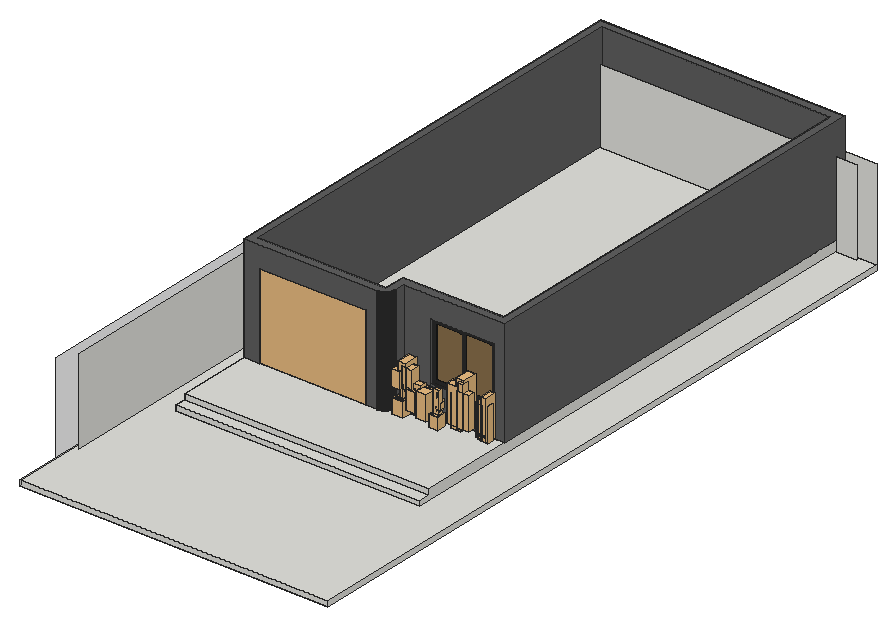
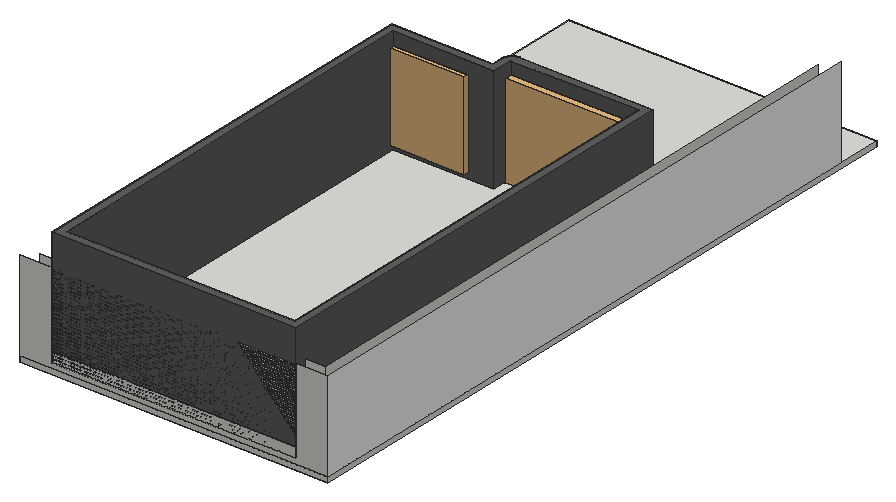
# SketchUp Ruby script. Lengths in inches.
U = 1.inch
M = Sketchup.active_model
def pt(a) = Geom::Point3d.new(a.map { |v| v * U })
def face(e, loops, mat)
  f = e.add_face(loops[0].map { |a| pt(a) })
  loops[1..].each { |l| e.add_face(l.map { |a| pt(a) }).erase! }
  f.material = f.back_material = mat if mat
  f
end
# faces: each face lists its corners as indices into pts; further lists are holes
def faces(e, pts, list, mat = nil) = list.each { |f| face(e, (f[0].is_a?(Array) ? f : [f]).map { |l| l.map { |i| pts[i] } }, mat) }
# xy, xz, yz: faces in a plane at the given z, y or x. An outline is a flat list of corners, or four numbers for a rectangle; further outlines are holes
def ring(l) = l.size == 4 ? [[l[0], l[1]], [l[2], l[1]], [l[2], l[3]], [l[0], l[3]]] : l.each_slice(2).to_a
def flat(e, list, mat, &to3) = list.each { |f| face(e, (f[0].is_a?(Array) ? f : [f]).map { |l| ring(l).map { |u, v| to3.(u, v) } }, mat) }
def xy(e, z, list, mat = nil) = flat(e, list, mat) { |x, y| [x, y, z] }
def xz(e, y, list, mat = nil) = flat(e, list, mat) { |x, z| [x, y, z] }
def yz(e, x, list, mat = nil) = flat(e, list, mat) { |y, z| [x, y, z] }
def lines(e, pts, list) = list.each { |a, b| e.add_line(pt(pts[a]), pt(pts[b])) }
# prism: a flat outline (further loops are holes) pulled along v
def prism(e, loops, v, mat = nil)
  f = face(e, loops, mat); d = Geom::Vector3d.new(v.map { |x| x * U })
  f.pushpull(f.normal.samedirection?(d) ? d.length : -d.length)
end
def box(e, o, s, mat = nil) = prism(e, [[o, [o[0] + s[0], o[1], o[2]], [o[0] + s[0], o[1] + s[1], o[2]], [o[0], o[1] + s[1], o[2]]]], [0, 0, s[2]], mat)
def at(x, y, z, deg = 0) = Geom::Transformation.translation(pt([x, y, z])) * Geom::Transformation.rotation(ORIGIN, Z_AXIS, deg.degrees)
def axes(o, x, y, z) = Geom::Transformation.new([*x, 0, *y, 0, *z, 0, *pt(o).to_a, 1])
def part(name) = M.definitions.add(name)
# library, detail: a bought-in or finely detailed component or shape, given as its bounding box
def library(name, o, s) = part(name).tap { |d| box(d.entities, o, s) }
def detail(e, o, s) = box(e.add_group.entities, o, s)
def put(e, d, t, mat = nil) = e.add_instance(d, t).tap { |i| i.material = mat if mat }
def group(e, t, mat = nil) = e.add_group.tap { |g| g.transformation = t; g.material = mat if mat }.entities
root = M.entities
M.materials.add("1421 AP 8232 ELEGANT GREY").color = [96, 96, 96]
M.materials.add("BANANA_BIG_STVOL_1").color = [93, 83, 53]
M.materials.add("Glass_Tinted_Gray").color = [0, 0, 0]
M.materials["Glass_Tinted_Gray"].alpha = 0.125
M.materials.add("POT_TEXTURE_2").color = [160, 154, 144]
M.materials.add("[0135_DarkGray]").color = [81, 81, 81]
M.materials.add("[Metal Seamed]").color = [36, 36, 35]
M.materials.add("[Mirror 02]").color = [229, 229, 229]
M.materials.add("[Quartz Light Grey]").color = [251, 251, 252]
M.materials.add("[Terrazzo Light Blue]").color = [196, 214, 227]
M.materials.add("soil1").color = [68, 55, 47]
M.materials.add("white_concrete_pot1").color = [212, 211, 204]
M.materials.add("wood_1").color = [140, 119, 94]
c1 = library("Group\#110",[-310.7,1952.62,354.63],[79.53,58.52,39.48])
c2 = library("Group\#213",[-330.26,-2159.14,612.04],[116.66,119.22,673.97])
c3 = library("Group\#85",[-312.76,2118.02,370.79],[80.37,61.43,57.53])
c4 = library("Group\#192",[-513.94,-1201.2,195.17],[480.66,557.42,1160.08])
c5 = library("Group\#163",[-447.02,-464.95,536.35],[343.73,346.24,39.39])
c6 = library("Group\#189",[-492.14,-508.4,-4.15],[433.72,431.71,567.03])
c7 = library("Group\#129",[-315.77,2202.04,371],[80.74,54.44,37.85])
c8 = library("Group\#206",[-390.1,-1177.12,195.59],[220.93,265.44,790.12])
c9 = library("Group\#210",[-480.3,-2300.47,677.45],[398.14,398.43,28.25])
c10 = library("Group\#217",[-568.09,-2386.9,-3.76],[573.62,569.18,700.28])
c11 = library("Group\#160",[-455.56,899.32,410.78],[341.21,610.33,1581.5])
c12 = library("Group\#104",[-330.83,2117.69,370.2],[61.83,80.2,35.55])
c13 = library("Group\#109",[-340.96,1970.4,361.28],[81.22,51.59,61.62])
c14 = library("Group\#154",[-445.29,890.31,329.28],[284.3,304.08,2023.29])
c15 = library("Group\#188",[-385.21,-446.52,494.02],[160.93,321.12,1142.36])
c16 = library("Group\#173",[-341.93,-403.49,744.8125],[64.83,96.32,132.15])
c17 = library("Group\#205",[-445.7,-1606.55,154.18],[255.44,283.57,849.28])
c18 = library("Group\#120",[-363.89,1895.22,354.63],[76.92,66.54,39.48])
c19 = library("Group\#135",[-366.3125,2177.8,359.41],[79.9,61.23,37.86])
c20 = library("Group\#186",[-422.77,-235.4,843.61],[178.54,197.77,233.54])
c21 = library("Group\#131",[-372.4375,2154.5,374],[76.125,67.08,39.0625])
c22 = library("Group\#102",[-362.86,1963.26,351.01],[55.56,80.44,37.9])
c23 = library("Group\#193",[-545.36,-1775.03,287.125],[412.21,432,920.68])
c24 = library("Group\#177",[-388.93,-514.39,838.93],[89.79,77.73,82.08])
c25 = library("Group\#174",[-424,-312.27,817.53],[158.81,108.06,136.45])
c26 = library("Group\#96",[-374.28,1979.7,369.99],[51.81,82.66,37.9])
c27 = library("Group\#164",[-394.9,-448.99,911.74],[90.19,96.88,85.93])
c28 = library("Group\#121",[-390.04,2074.71,363.78],[77.3,84.83,61.55])
c29 = library("Group\#94",[-392.38,2142.99,345.23],[79.77,60.6,39.05])
c30 = library("Group\#167",[-438.92,-265.61,702.3],[171.52,146.16,133.5])
c31 = library("Group\#98",[-389.63,2051.04,359.41],[56.81,81.38,37.86])
c32 = library("Group\#127",[-397.18,1916.74,372.44],[70.02,74.57,49.25])
c33 = library("Group\#219",[-550.09,-2664.39,1031.96],[371.42,533.86,798])
c34 = library("Group\#178",[-409.02,-515.05,915.53],[69.62,77.27,65.47])
c35 = library("Group\#122",[-419.21,1941.11,355.02],[73.1,71.21,39.06])
c36 = library("Group\#143",[-527.15,2088.47,150.96],[267.01,328.12,1599.25])
c37 = library("Group\#169",[-545.09,-386.51,922.3125],[300.25,219.65,227.33])
c38 = library("Group\#95",[-433.57,2042.61,369.7],[71.79,72.8,37.85])
c39 = library("Group\#97",[-432.01,1984.38,372.6875],[64.1,75.95,39.0625])
c40 = library("Group\#101",[-435.875,2067.96,347.82],[58.32,80.53,38.29])
c41 = library("Group\#176",[-568.91,-444.37,1285.4],[307.6,179.39,277.93])
c42 = library("Group\#140",[-571.16,1736.08,232.33],[294.08,306.57,1438.75])
c43 = library("Group\#180",[-498.98,-524.4,908.45],[120.83,107.95,112.98])
c44 = library("Group\#197",[-640.625,-1318.37,287.11],[396.64,314.81,689.96])
c45 = library("Group\#148",[-616.67,2098.6,178.29],[331.19,111.16,1177.92])
c46 = library("Group\#214",[-667.53,-2111.4375,1071.74],[420.02,555.28,968.03])
c47 = library("Group\#200",[-619.83,-1636.3,288.9],[316.15,456.61,1171.28])
c48 = library("Group\#159",[-662.41,217.3,320.04],[397.32,658.3,1732.06])
c49 = library("Group\#144",[-675.58,1862.05,152.55],[378.81,196.01,1743.84])
c50 = library("Group\#157",[-733.48,439.625,202.64],[456.28,533.12,1536.78])
c51 = library("Group\#150",[-792.12,2067.32,152.13],[549.56,259.52,1931.8])
c52 = library("Group\#201",[-738.91,-1210.08,301],[426.4,388.88,1000.79])
c53 = library("Group\#198",[-750.24,-1478.51,301.56],[423.84,451.05,998.69])
c54 = library("Group\#138",[-904.81,1865.01,156.3],[624.43,217.34,1227.7])
c55 = library("Group\#216",[-943.22,-2312.1875,967.59],[670.63,402.45,1245.73])
c56 = library("Group\#156",[-1038.76,656.55,345.34],[733.18,460.51,2065.7])
c57 = library("Curtain assembly",[0,0,0],[57.48,5.46,98.43])
c58 = library("Curtains",[0,0,0],[121.73,8.19,117.22])
c59 = library("Group\#3",[0,-4.26,0],[120,5.53,96])
c60 = part("PENTEK_RP Fineline 50S_Sliding_DoorCase_E1")
box(c60.entities,[0,0,0],[1.51,3.66,99.27],"[0135_DarkGray]")
c61 = part("PENTEK_RP Fineline 50S_SlidingDooe_Case_E2")
box(c61.entities,[0,0,0],[96.25,3.66,1.51],"[0135_DarkGray]")
c62 = part("pentek_RP Fineline 50S_SlidingDoor_Case")
put(c62.entities,c60,at(97.76,0,0))
put(c62.entities,c61,at(1.51,0,0))
put(c62.entities,c60,at(0,0,0),"[Metal Seamed]")
put(c62.entities,c61,at(1.51,0,97.76),"[Metal Seamed]")
c63 = part("PENTEK_RP Fineline 50S_SlidingDoor_GlazingBead_2")
box(c63.entities,[0,0,0],[0.56,0.59,94.39],"[0135_DarkGray]")
c64 = part("PENTEK_RP Fineline 50S_SlidingDoor_Glass")
box(c64.entities,[0,0,0],[46.58,0.16,94.39],"Glass_Tinted_Gray")
c65 = part("PENTEK_RP Fineline 50S_SlidingDoor_GlazingBead")
box(c65.entities,[0,0,0],[45.47,0.59,0.56],"[0135_DarkGray]")
c66 = part("PENTEK_RP Fineline 50S_SlidingDoor_Leaf_E1")
xy(c66.entities,0,[[0,0,0.93,1.97],[0.93,1.57,1.49,1.97]],"[0135_DarkGray]")
xy(c66.entities,96.25,[[0,0,0.93,0,0.93,1.57,1.49,1.57,1.49,1.97,0,1.97]],"[0135_DarkGray]")
xz(c66.entities,0,[[0,0,0.93,96.25]],"[0135_DarkGray]")
xz(c66.entities,1.57,[[0.93,0,1.49,95.32],[0.93,95.32,1.49,96.25]],"[0135_DarkGray]")
xz(c66.entities,1.97,[[0,0,1.49,96.25]],"[0135_DarkGray]")
yz(c66.entities,0,[[0,0,1.97,96.25]],"[0135_DarkGray]")
yz(c66.entities,0.93,[[0,0,1.57,0.93],[0,0.93,1.57,95.32],[0,95.32,1.57,96.25]],"[0135_DarkGray]")
yz(c66.entities,1.49,[[1.57,0,1.97,95.32],[1.57,95.32,1.97,96.25]],"[0135_DarkGray]")
c67 = part("PENTEK_RP Fineline 50S_SlidingDoor_Leaf_E2")
xy(c67.entities,0,[[0,0,0,1.57,0.56,1.57,0.56,1.97,46.02,1.97,46.02,1.57,46.58,1.57,46.58,0]],"[0135_DarkGray]")
xy(c67.entities,0.93,[[0,0,46.58,1.57]],"[0135_DarkGray]")
xy(c67.entities,1.49,[[0.56,1.57,46.02,1.97]],"[0135_DarkGray]")
xz(c67.entities,0,[[0,0,46.58,0.93]],"[0135_DarkGray]")
xz(c67.entities,1.57,[[0,0,0.56,0.93],[46.02,0,46.58,0.93],[0.56,0.93,46.02,1.49]],"[0135_DarkGray]")
xz(c67.entities,1.97,[[0.56,0,46.02,1.49]],"[0135_DarkGray]")
yz(c67.entities,0,[[0,0,1.57,0.93]],"[0135_DarkGray]")
yz(c67.entities,0.56,[[1.57,0,1.97,0.93],[1.57,0.93,1.97,1.49]],"[0135_DarkGray]")
yz(c67.entities,46.02,[[1.57,0,1.97,0.93],[1.57,0.93,1.97,1.49]],"[0135_DarkGray]")
yz(c67.entities,46.58,[[0,0,1.57,0.93]],"[0135_DarkGray]")
c68 = part("PENTEK_RP Fineline S_SlidingDoor_Leaf1")
put(c68.entities,c63,at(0.93,0,0.93))
put(c68.entities,c63,at(46.96,0,0.93))
put(c68.entities,c64,at(1.49,1.42,0.93))
put(c68.entities,c65,at(1.49,0,0.93))
put(c68.entities,c64,at(1.49,0.59,0.93),"[Terrazzo Light Blue]")
put(c68.entities,c66,at(0,0,0))
put(c68.entities,c66,axes([48.44,0,0],[-1,0,0],[0,1,0],[0,0,1]))
put(c68.entities,c67,axes([0.93,0,96.25],[1,0,0],[0,1,0],[0,0,-1]))
put(c68.entities,c67,at(0.93,0,0))
put(c68.entities,c65,at(1.49,0,94.77))
c69 = part("PENTEK_RP Fineline 50S_SlidingDoor_Leaf2")
put(c69.entities,c64,at(1.49,1.42,0.93))
put(c69.entities,c65,at(1.49,0,94.77))
put(c69.entities,c63,at(46.96,0,0.93))
put(c69.entities,c64,at(1.49,0.59,0.93),"[Mirror 02]")
put(c69.entities,c63,at(0.93,0,0.93))
put(c69.entities,c66,at(0,0,0))
put(c69.entities,c66,axes([48.44,0,0],[-1,0,0],[0,1,0],[0,0,1]))
put(c69.entities,c65,at(1.49,0,0.93))
put(c69.entities,c67,axes([0.93,0,96.25],[1,0,0],[0,1,0],[0,0,-1]))
put(c69.entities,c67,at(0.93,0,0))
c70 = part("PENTEK - Slimmest Steel Sliding Door / Window\#1")
put(c70.entities,c62,at(0,-1.88,-0.09))
put(c70.entities,c68,at(1.51,-2.27,1.42))
put(c70.entities,c69,at(49.32,-0.3,1.42))
xz(root,763,[[12,-12,336,84]])
xz(root,775,[[0,-18,348,84]])
yz(root,0,[[50,-18,775,84]],"[Quartz Light Grey]")
yz(root,12,[[67,-12,763,84]])
put(root,c1,axes([253.68,273.14,0.11],[0,-0.02318,0],[0.02157,0,0],[0,0,0.02333]),"white_concrete_pot1")
put(root,c2,axes([253.68,273.14,0.11],[0,-0.02318,0],[0.02157,0,0],[0,0,0.02333]),"BANANA_BIG_STVOL_1")
put(root,c3,axes([253.68,273.14,0.11],[0,-0.02318,0],[0.02157,0,0],[0,0,0.02333]),"white_concrete_pot1")
put(root,c4,axes([253.68,273.14,0.11],[0,-0.02318,0],[0.02157,0,0],[0,0,0.02333]))
put(root,c5,axes([253.68,273.14,0.11],[0,-0.02318,0],[0.02157,0,0],[0,0,0.02333]),"soil1")
put(root,c6,axes([253.68,273.14,0.11],[0,-0.02318,0],[0.02157,0,0],[0,0,0.02333]),"POT_TEXTURE_2")
put(root,c7,axes([253.68,273.14,0.11],[0,-0.02318,0],[0.02157,0,0],[0,0,0.02333]),"white_concrete_pot1")
g1 = group(root,at(253.68,273.14,0.11),"white_concrete_pot1")
detail(g1,[40.58,5.65,8.19],[1.57,1.63,0.87])
put(root,c8,axes([253.68,273.14,0.11],[0,-0.02318,0],[0.02157,0,0],[0,0,0.02333]))
put(root,c9,axes([253.68,273.14,0.11],[0,-0.02318,0],[0.02157,0,0],[0,0,0.02333]),"soil1")
put(root,c10,axes([253.68,273.14,0.11],[0,-0.02318,0],[0.02157,0,0],[0,0,0.02333]),"POT_TEXTURE_2")
g2 = group(root,at(253.68,273.14,0.11),"white_concrete_pot1")
detail(g2,[44.84,5.64,7.91],[1.49,1.76,0.92])
put(root,c11,axes([253.68,273.14,0.11],[0,-0.02318,0],[0.02157,0,0],[0,0,0.02333]))
put(root,c12,axes([253.68,273.14,0.11],[0,-0.02318,0],[0.02157,0,0],[0,0,0.02333]),"white_concrete_pot1")
put(root,c13,axes([253.68,273.14,0.11],[0,-0.02318,0],[0.02157,0,0],[0,0,0.02333]),"white_concrete_pot1")
g3 = group(root,at(253.68,273.14,0.11),"white_concrete_pot1")
detail(g3,[40.82,6.3,8.64],[1.71,1.42,0.87])
put(root,c14,axes([253.68,273.14,0.11],[0,-0.02318,0],[0.02157,0,0],[0,0,0.02333]))
put(root,c15,axes([253.68,273.14,0.11],[0,-0.02318,0],[0.02157,0,0],[0,0,0.02333]),"wood_1")
put(root,c16,axes([253.68,273.14,0.11],[0,-0.02318,0],[0.02157,0,0],[0,0,0.02333]))
put(root,c17,axes([253.68,273.14,0.11],[0,-0.02318,0],[0.02157,0,0],[0,0,0.02333]))
put(root,c18,axes([253.68,273.14,0.11],[0,-0.02318,0],[0.02157,0,0],[0,0,0.02333]),"white_concrete_pot1")
put(root,c19,axes([253.68,273.14,0.11],[0,-0.02318,0],[0.02157,0,0],[0,0,0.02333]),"white_concrete_pot1")
put(root,c20,axes([253.68,273.14,0.11],[0,-0.02318,0],[0.02157,0,0],[0,0,0.02333]))
put(root,c21,axes([253.68,273.14,0.11],[0,-0.02318,0],[0.02157,0,0],[0,0,0.02333]),"white_concrete_pot1")
put(root,c22,axes([253.68,273.14,0.11],[0,-0.02318,0],[0.02157,0,0],[0,0,0.02333]),"white_concrete_pot1")
put(root,c23,axes([253.68,273.14,0.11],[0,-0.02318,0],[0.02157,0,0],[0,0,0.02333]))
put(root,c24,axes([253.68,273.14,0.11],[0,-0.02318,0],[0.02157,0,0],[0,0,0.02333]))
put(root,c25,axes([253.68,273.14,0.11],[0,-0.02318,0],[0.02157,0,0],[0,0,0.02333]))
put(root,c26,axes([253.68,273.14,0.11],[0,-0.02318,0],[0.02157,0,0],[0,0,0.02333]),"white_concrete_pot1")
put(root,c27,axes([253.68,273.14,0.11],[0,-0.02318,0],[0.02157,0,0],[0,0,0.02333]))
put(root,c28,axes([253.68,273.14,0.11],[0,-0.02318,0],[0.02157,0,0],[0,0,0.02333]),"white_concrete_pot1")
put(root,c29,axes([253.68,273.14,0.11],[0,-0.02318,0],[0.02157,0,0],[0,0,0.02333]),"white_concrete_pot1")
put(root,c30,axes([253.68,273.14,0.11],[0,-0.02318,0],[0.02157,0,0],[0,0,0.02333]))
g4 = group(root,at(253.68,273.14,0.11),"white_concrete_pot1")
detail(g4,[43.93,7.3,8.4],[1.4,1.85,0.87])
put(root,c31,axes([253.68,273.14,0.11],[0,-0.02318,0],[0.02157,0,0],[0,0,0.02333]),"white_concrete_pot1")
put(root,c32,axes([253.68,273.14,0.11],[0,-0.02318,0],[0.02157,0,0],[0,0,0.02333]),"white_concrete_pot1")
put(root,c33,axes([253.68,273.14,0.11],[0,-0.02318,0],[0.02157,0,0],[0,0,0.02333]))
put(root,c34,axes([253.68,273.14,0.11],[0,-0.02318,0],[0.02157,0,0],[0,0,0.02333]))
put(root,c35,axes([253.68,273.14,0.11],[0,-0.02318,0],[0.02157,0,0],[0,0,0.02333]),"white_concrete_pot1")
g5 = group(root,at(253.68,273.14,0.11),"white_concrete_pot1")
detail(g5,[45.57,8.17,8.63],[1.72,1.51,0.89])
put(root,c36,axes([253.68,273.14,0.11],[0,-0.02318,0],[0.02157,0,0],[0,0,0.02333]))
put(root,c37,axes([253.68,273.14,0.11],[0,-0.02318,0],[0.02157,0,0],[0,0,0.02333]))
g6 = group(root,at(253.68,273.14,0.11),"white_concrete_pot1")
detail(g6,[43.74,8.27,8.18],[1.35,1.83,0.89])
put(root,c38,axes([253.68,273.14,0.11],[0,-0.02318,0],[0.02157,0,0],[0,0,0.02333]),"white_concrete_pot1")
put(root,c39,axes([253.68,273.14,0.11],[0,-0.02318,0],[0.02157,0,0],[0,0,0.02333]),"white_concrete_pot1")
put(root,c40,axes([253.68,273.14,0.11],[0,-0.02318,0],[0.02157,0,0],[0,0,0.02333]),"white_concrete_pot1")
put(root,c41,axes([253.68,273.14,0.11],[0,-0.02318,0],[0.02157,0,0],[0,0,0.02333]))
put(root,c42,axes([253.68,273.14,0.11],[0,-0.02318,0],[0.02157,0,0],[0,0,0.02333]))
put(root,c43,axes([253.68,273.14,0.11],[0,-0.02318,0],[0.02157,0,0],[0,0,0.02333]))
put(root,c44,axes([253.68,273.14,0.11],[0,-0.02318,0],[0.02157,0,0],[0,0,0.02333]))
put(root,c45,axes([253.68,273.14,0.11],[0,-0.02318,0],[0.02157,0,0],[0,0,0.02333]))
put(root,c46,axes([253.68,273.14,0.11],[0,-0.02318,0],[0.02157,0,0],[0,0,0.02333]))
put(root,c47,axes([253.68,273.14,0.11],[0,-0.02318,0],[0.02157,0,0],[0,0,0.02333]))
put(root,c48,axes([253.68,273.14,0.11],[0,-0.02318,0],[0.02157,0,0],[0,0,0.02333]))
put(root,c49,axes([253.68,273.14,0.11],[0,-0.02318,0],[0.02157,0,0],[0,0,0.02333]))
put(root,c50,axes([253.68,273.14,0.11],[0,-0.02318,0],[0.02157,0,0],[0,0,0.02333]))
put(root,c51,axes([253.68,273.14,0.11],[0,-0.02318,0],[0.02157,0,0],[0,0,0.02333]))
put(root,c52,axes([253.68,273.14,0.11],[0,-0.02318,0],[0.02157,0,0],[0,0,0.02333]))
put(root,c53,axes([253.68,273.14,0.11],[0,-0.02318,0],[0.02157,0,0],[0,0,0.02333]))
put(root,c54,axes([253.68,273.14,0.11],[0,-0.02318,0],[0.02157,0,0],[0,0,0.02333]))
put(root,c55,axes([253.68,273.14,0.11],[0,-0.02318,0],[0.02157,0,0],[0,0,0.02333]))
put(root,c56,axes([253.68,273.14,0.11],[0,-0.02318,0],[0.02157,0,0],[0,0,0.02333]))
g7 = group(root,at(0,0,-18))
box(g7,[0,0,-6],[348,775,6])
g8 = group(root,at(36,271,0))
prism(g8,[[[0,-84,0],[0,504,0],[0,504,-12],[0,-96,-12],[0,-96,-6],[0,-84,-6]]],[276,0,0])
g9 = group(root,at(36,295,0),"1421 AP 8232 ELEGANT GREY")
xy(g9,0,[[0,-24,0,480,276,480,276,0,162,0,162,-12.3125,161.99,-12.47,161.98,-12.63,161.97,-12.78,161.95,-13.1,161.93,-13.25,161.92,-13.41,161.9,-13.57,161.875,-13.72,161.85,-13.88,161.83,-14.03,161.8,-14.1875,161.77,-14.34,161.74,-14.49,161.7,-14.65,161.67,-14.8,161.63,-14.95,161.59,-15.11,161.51,-15.41,161.36,-15.86,161.3125,-16.01,161.26,-16.15,161.2,-16.3,161.15,-16.45,161.09,-16.59,161.03,-16.74,160.96,-16.88,160.9,-17.02,160.83,-17.17,160.55,-17.73,160.47,-17.86,160.39,-18,160.3125,-18.14,160.23,-18.27,160.15,-18.4,160.0625,-18.54,159.98,-18.67,159.8,-18.93,159.71,-19.05,159.62,-19.18,159.52,-19.31,159.42,-19.43,159.33,-19.55,159.23,-19.67,159.02,-19.91,158.92,-20.03,158.8125,-20.15,158.7,-20.26,158.6,-20.375,158.49,-20.49,158.375,-20.6,158.26,-20.7,158.15,-20.8125,158.03,-20.92,157.91,-21.02,157.67,-21.23,157.55,-21.33,157.43,-21.42,157.31,-21.52,157.18,-21.62,157.05,-21.71,156.93,-21.8,156.67,-21.98,156.54,-22.0625,156.4,-22.15,156.27,-22.23,156.14,-22.3125,156,-22.39,155.86,-22.47,155.73,-22.55,155.17,-22.83,155.02,-22.9,154.88,-22.96,154.74,-23.03,154.59,-23.09,154.45,-23.15,154.3,-23.2,154.15,-23.26,154.01,-23.3125,153.86,-23.36,153.41,-23.51,153.11,-23.59,152.95,-23.63,152.8,-23.67,152.65,-23.7,152.49,-23.74,152.34,-23.77,152.1875,-23.8,152.03,-23.83,151.88,-23.85,151.72,-23.875,151.57,-23.9,151.41,-23.92,151.25,-23.93,151.1,-23.95,150.78,-23.97,150.63,-23.98,150.47,-23.99,150.3125,-24,138,-24,138,-15,153,-15,153,9,267,9,267,471,9,471,9,-15,18,-15,18,-24]])
xy(g9,30,[[192,0,264,9]])
xy(g9,96,[[18,-24,138,-15],[192,0,264,9]])
xy(g9,120,[[[0,-24,150.3125,-24,150.47,-23.99,150.63,-23.98,150.78,-23.97,151.1,-23.95,151.25,-23.93,151.41,-23.92,151.57,-23.9,151.72,-23.875,151.88,-23.85,152.03,-23.83,152.1875,-23.8,152.34,-23.77,152.49,-23.74,152.65,-23.7,152.8,-23.67,152.95,-23.63,153.11,-23.59,153.41,-23.51,153.86,-23.36,154.01,-23.3125,154.15,-23.26,154.3,-23.2,154.45,-23.15,154.59,-23.09,154.74,-23.03,154.88,-22.96,155.02,-22.9,155.17,-22.83,155.73,-22.55,155.86,-22.47,156,-22.39,156.14,-22.3125,156.27,-22.23,156.4,-22.15,156.54,-22.0625,156.67,-21.98,156.93,-21.8,157.05,-21.71,157.18,-21.62,157.31,-21.52,157.43,-21.42,157.55,-21.33,157.67,-21.23,157.91,-21.02,158.03,-20.92,158.15,-20.8125,158.26,-20.7,158.375,-20.6,158.49,-20.49,158.6,-20.375,158.7,-20.26,158.8125,-20.15,158.92,-20.03,159.02,-19.91,159.23,-19.67,159.33,-19.55,159.42,-19.43,159.52,-19.31,159.62,-19.18,159.71,-19.05,159.8,-18.93,159.98,-18.67,160.0625,-18.54,160.15,-18.4,160.23,-18.27,160.3125,-18.14,160.39,-18,160.47,-17.86,160.55,-17.73,160.83,-17.17,160.9,-17.02,160.96,-16.88,161.03,-16.74,161.09,-16.59,161.15,-16.45,161.2,-16.3,161.26,-16.15,161.3125,-16.01,161.36,-15.86,161.51,-15.41,161.59,-15.11,161.63,-14.95,161.67,-14.8,161.7,-14.65,161.74,-14.49,161.77,-14.34,161.8,-14.1875,161.83,-14.03,161.85,-13.88,161.875,-13.72,161.9,-13.57,161.92,-13.41,161.93,-13.25,161.95,-13.1,161.97,-12.78,161.98,-12.63,161.99,-12.47,162,-12.3125,162,0,276,0,276,480,0,480],[9,-15,9,471,267,471,267,9,153,9,153,-15]]])
xz(g9,-24,[[0,0,18,0,18,96,138,96,138,0,150,0,150,120,0,120],[150,0,150.16,120],[150.16,0,150.3125,120]])
xz(g9,-15,[[9,0,9,120,153,120,153,0,138,0,138,96,18,96,18,0]])
xz(g9,0,[[[162,0,276,120],[192,30,264,96]]])
xz(g9,9,[[[153,0,267,120],[192,30,264,96]]])
xz(g9,471,[[9,0,267,120]])
xz(g9,480,[[0,0,276,120]])
yz(g9,0,[[-24,0,480,120]])
yz(g9,9,[[-15,0,471,120]])
yz(g9,18,[[-24,0,-15,96]])
yz(g9,138,[[-24,0,-15,96]])
yz(g9,153,[[-15,0,9,120]])
yz(g9,162,[[-12.3125,0,-12.16,120],[-12.16,0,-12,120],[-12,0,0,120]])
yz(g9,192,[[0,30,9,96]])
yz(g9,264,[[0,30,9,96]])
yz(g9,267,[[9,0,471,120]])
yz(g9,276,[[0,0,480,120]])
p = [[150.47,-23.99,120],[150.3125,-24,120],[150.3125,-24,0],[150.47,-23.99,0],[150.63,-23.98,120],[150.63,-23.98,0],
  [150.78,-23.97,120],[150.78,-23.97,0],[150.94,-23.96,120],[150.94,-23.96,0],[151.1,-23.95,120],[151.1,-23.95,0],
  [151.25,-23.93,120],[151.25,-23.93,0],[151.41,-23.92,120],[151.41,-23.92,0],[151.57,-23.9,120],[151.57,-23.9,0],
  [151.72,-23.875,120],[151.72,-23.875,0],[151.88,-23.85,120],[151.88,-23.85,0],[152.03,-23.83,120],[152.03,-23.83,0],
  [152.1875,-23.8,120],[152.1875,-23.8,0],[152.34,-23.77,120],[152.34,-23.77,0],[152.49,-23.74,120],[152.49,-23.74,0],
  [152.65,-23.7,120],[152.65,-23.7,0],[152.8,-23.67,120],[152.8,-23.67,0],[152.95,-23.63,120],[152.95,-23.63,0],
  [153.11,-23.59,120],[153.11,-23.59,0],[153.26,-23.55,120],[153.26,-23.55,0],[153.41,-23.51,120],[153.41,-23.51,0],
  [153.56,-23.46,120],[153.56,-23.46,0],[153.71,-23.41,120],[153.71,-23.41,0],[153.86,-23.36,120],[153.86,-23.36,0],
  [154.01,-23.3125,120],[154.01,-23.3125,0],[154.15,-23.26,120],[154.15,-23.26,0],[154.3,-23.2,120],[154.3,-23.2,0],
  [154.45,-23.15,120],[154.45,-23.15,0],[154.59,-23.09,120],[154.59,-23.09,0],[154.74,-23.03,120],[154.74,-23.03,0],
  [154.88,-22.96,120],[154.88,-22.96,0],[155.02,-22.9,120],[155.02,-22.9,0],[155.17,-22.83,120],[155.17,-22.83,0],
  [155.31,-22.76,120],[155.31,-22.76,0],[155.45,-22.69,120],[155.45,-22.69,0],[155.59,-22.62,120],[155.59,-22.62,0],
  [155.73,-22.55,120],[155.73,-22.55,0],[155.86,-22.47,120],[155.86,-22.47,0],[156,-22.39,120],[156,-22.39,0],
  [156.14,-22.3125,120],[156.14,-22.3125,0],[156.27,-22.23,120],[156.27,-22.23,0],[156.4,-22.15,120],[156.4,-22.15,0],
  [156.54,-22.0625,120],[156.54,-22.0625,0],[156.67,-21.98,120],[156.67,-21.98,0],[156.8,-21.89,120],[156.8,-21.89,0],
  [156.93,-21.8,120],[156.93,-21.8,0],[157.05,-21.71,120],[157.05,-21.71,0],[157.18,-21.62,120],[157.18,-21.62,0],
  [157.31,-21.52,120],[157.31,-21.52,0],[157.43,-21.42,120],[157.43,-21.42,0],[157.55,-21.33,120],[157.55,-21.33,0],
  [157.67,-21.23,120],[157.67,-21.23,0],[157.79,-21.125,120],[157.79,-21.125,0],[157.91,-21.02,120],[157.91,-21.02,0],
  [158.03,-20.92,120],[158.03,-20.92,0],[158.15,-20.8125,120],[158.15,-20.8125,0],[158.26,-20.7,120],[158.26,-20.7,0],
  [158.375,-20.6,120],[158.375,-20.6,0],[158.49,-20.49,120],[158.49,-20.49,0],[158.6,-20.375,120],[158.6,-20.375,0],
  [158.7,-20.26,120],[158.7,-20.26,0],[158.8125,-20.15,120],[158.8125,-20.15,0],[158.92,-20.03,120],[158.92,-20.03,0],
  [159.02,-19.91,120],[159.02,-19.91,0],[159.125,-19.79,120],[159.125,-19.79,0],[159.23,-19.67,120],[159.23,-19.67,0],
  [159.33,-19.55,120],[159.33,-19.55,0],[159.42,-19.43,120],[159.42,-19.43,0],[159.52,-19.31,120],[159.52,-19.31,0],
  [159.62,-19.18,120],[159.62,-19.18,0],[159.71,-19.05,120],[159.71,-19.05,0],[159.8,-18.93,120],[159.8,-18.93,0],
  [159.89,-18.8,120],[159.89,-18.8,0],[159.98,-18.67,120],[159.98,-18.67,0],[160.0625,-18.54,120],[160.0625,-18.54,0],
  [160.15,-18.4,120],[160.15,-18.4,0],[160.23,-18.27,120],[160.23,-18.27,0],[160.3125,-18.14,120],[160.3125,-18.14,0],
  [160.39,-18,120],[160.39,-18,0],[160.47,-17.86,120],[160.47,-17.86,0],[160.55,-17.73,120],[160.55,-17.73,0],
  [160.62,-17.59,120],[160.62,-17.59,0],[160.69,-17.45,120],[160.69,-17.45,0],[160.76,-17.31,120],[160.76,-17.31,0],
  [160.83,-17.17,120],[160.83,-17.17,0],[160.9,-17.02,120],[160.9,-17.02,0],[160.96,-16.88,120],[160.96,-16.88,0],
  [161.03,-16.74,120],[161.03,-16.74,0],[161.09,-16.59,120],[161.09,-16.59,0],[161.15,-16.45,120],[161.15,-16.45,0],
  [161.2,-16.3,120],[161.2,-16.3,0],[161.26,-16.15,120],[161.26,-16.15,0],[161.3125,-16.01,120],[161.3125,-16.01,0],
  [161.36,-15.86,120],[161.36,-15.86,0],[161.41,-15.71,120],[161.41,-15.71,0],[161.46,-15.56,120],[161.46,-15.56,0],
  [161.51,-15.41,120],[161.51,-15.41,0],[161.55,-15.26,120],[161.55,-15.26,0],[161.59,-15.11,120],[161.59,-15.11,0],
  [161.63,-14.95,120],[161.63,-14.95,0],[161.67,-14.8,120],[161.67,-14.8,0],[161.7,-14.65,120],[161.7,-14.65,0],
  [161.74,-14.49,120],[161.74,-14.49,0],[161.77,-14.34,120],[161.77,-14.34,0],[161.8,-14.1875,120],[161.8,-14.1875,0],
  [161.83,-14.03,120],[161.83,-14.03,0],[161.85,-13.88,120],[161.85,-13.88,0],[161.875,-13.72,120],[161.875,-13.72,0],
  [161.9,-13.57,120],[161.9,-13.57,0],[161.92,-13.41,120],[161.92,-13.41,0],[161.93,-13.25,120],[161.93,-13.25,0],
  [161.95,-13.1,120],[161.95,-13.1,0],[161.96,-12.94,120],[161.96,-12.94,0],[161.97,-12.78,120],[161.97,-12.78,0],
  [161.98,-12.63,120],[161.98,-12.63,0],[161.99,-12.47,120],[161.99,-12.47,0],[162,-12.3125,120],[162,-12.3125,0],
  [18,-24,0],[138,-24,0]]
faces(g9,p,[[0,1,2,3],[4,0,3,5],[6,4,5,7],[8,6,7,9],[10,8,9,11],[12,10,11,13],[14,12,13,15],[16,14,15,17],
  [18,16,17,19],[20,18,19,21],[22,20,21,23],[24,22,23,25],[26,24,25,27],[28,26,27,29],[30,28,29,31],[32,30,31,33],
  [34,32,33,35],[36,34,35,37],[38,36,37,39],[40,38,39,41],[42,40,41,43],[44,42,43,45],[46,44,45,47],[48,46,47,49],
  [50,48,49,51],[52,50,51,53],[54,52,53,55],[56,54,55,57],[58,56,57,59],[60,58,59,61],[62,60,61,63],[64,62,63,65],
  [66,64,65,67],[68,66,67,69],[70,68,69,71],[72,70,71,73],[74,72,73,75],[76,74,75,77],[78,76,77,79],[80,78,79,81],
  [82,80,81,83],[84,82,83,85],[86,84,85,87],[88,86,87,89],[90,88,89,91],[92,90,91,93],[94,92,93,95],[96,94,95,97],
  [98,96,97,99],[100,98,99,101],[102,100,101,103],[104,102,103,105],[106,104,105,107],[108,106,107,109],[110,108,109,111],[112,110,111,113],
  [114,112,113,115],[116,114,115,117],[118,116,117,119],[120,118,119,121],[122,120,121,123],[124,122,123,125],[126,124,125,127],[128,126,127,129],
  [130,128,129,131],[132,130,131,133],[134,132,133,135],[136,134,135,137],[138,136,137,139],[140,138,139,141],[142,140,141,143],[144,142,143,145],
  [146,144,145,147],[148,146,147,149],[150,148,149,151],[152,150,151,153],[154,152,153,155],[156,154,155,157],[158,156,157,159],[160,158,159,161],
  [162,160,161,163],[164,162,163,165],[166,164,165,167],[168,166,167,169],[170,168,169,171],[172,170,171,173],[174,172,173,175],[176,174,175,177],
  [178,176,177,179],[180,178,179,181],[182,180,181,183],[184,182,183,185],[186,184,185,187],[188,186,187,189],[190,188,189,191],[192,190,191,193],
  [194,192,193,195],[196,194,195,197],[198,196,197,199],[200,198,199,201],[202,200,201,203],[204,202,203,205],[206,204,205,207],[208,206,207,209],
  [210,208,209,211],[212,210,211,213],[214,212,213,215],[216,214,215,217],[218,216,217,219],[220,218,219,221],[222,220,221,223],[224,222,223,225],
  [226,224,225,227],[228,226,227,229],[230,228,229,231],[232,230,231,233]])
lines(g9,p,[[234,235]])
put(g9,c57,axes([183.08,9,6.8125],[1.46,0,0],[0,1,0],[0,0,1]))
put(g9,c58,axes([9,-6.81,0],[1.18298,0,0],[0,-1,0],[0,0,0.9]))
put(g9,c59,at(18,-19,0),"[Metal Seamed]")
g10 = group(g9,at(192,4.5,30),"[Metal Seamed]")
prism(g10,[[[72,0,0],[0,0,0],[0,0,66],[72,0,66]],[[70,0,64],[2,0,64],[2,0,2],[70,0,2]]],[0,-3,0])
put(g10,c70,axes([2,-1.59,2.06],[0.68498,0,0],[0,0.62,0],[0,0,0.62454]),"[Metal Seamed]")
